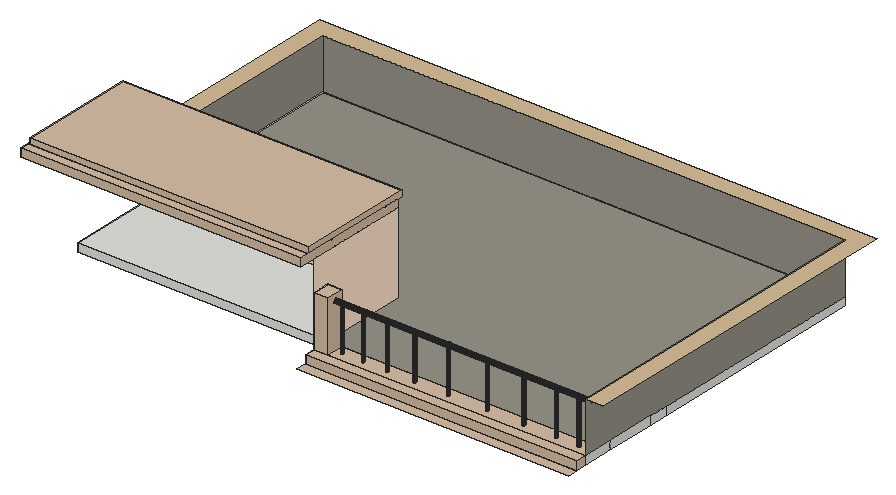
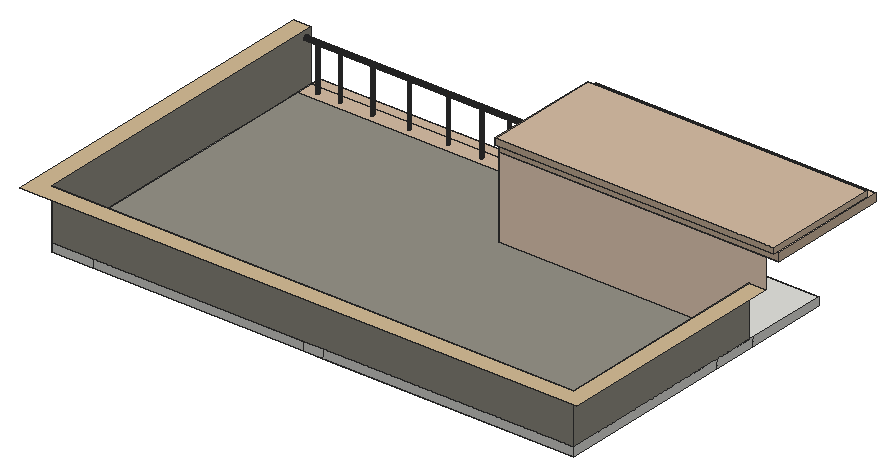
# SketchUp Ruby script. Lengths in inches.
U = 1.inch
M = Sketchup.active_model
def pt(a) = Geom::Point3d.new(a.map { |v| v * U })
def face(e, loops, mat)
  f = e.add_face(loops[0].map { |a| pt(a) })
  loops[1..].each { |l| e.add_face(l.map { |a| pt(a) }).erase! }
  f.material = f.back_material = mat if mat
  f
end
# faces: each face lists its corners as indices into pts; further lists are holes
def faces(e, pts, list, mat = nil) = list.each { |f| face(e, (f[0].is_a?(Array) ? f : [f]).map { |l| l.map { |i| pts[i] } }, mat) }
# xy, xz, yz: faces in a plane at the given z, y or x. An outline is a flat list of corners, or four numbers for a rectangle; further outlines are holes
def ring(l) = l.size == 4 ? [[l[0], l[1]], [l[2], l[1]], [l[2], l[3]], [l[0], l[3]]] : l.each_slice(2).to_a
def flat(e, list, mat, &to3) = list.each { |f| face(e, (f[0].is_a?(Array) ? f : [f]).map { |l| ring(l).map { |u, v| to3.(u, v) } }, mat) }
def xy(e, z, list, mat = nil) = flat(e, list, mat) { |x, y| [x, y, z] }
def xz(e, y, list, mat = nil) = flat(e, list, mat) { |x, z| [x, y, z] }
def yz(e, x, list, mat = nil) = flat(e, list, mat) { |y, z| [x, y, z] }
def lines(e, pts, list) = list.each { |a, b| e.add_line(pt(pts[a]), pt(pts[b])) }
# prism: a flat outline (further loops are holes) pulled along v
def prism(e, loops, v, mat = nil)
  f = face(e, loops, mat); d = Geom::Vector3d.new(v.map { |x| x * U })
  f.pushpull(f.normal.samedirection?(d) ? d.length : -d.length)
end
def box(e, o, s, mat = nil) = prism(e, [[o, [o[0] + s[0], o[1], o[2]], [o[0] + s[0], o[1] + s[1], o[2]], [o[0], o[1] + s[1], o[2]]]], [0, 0, s[2]], mat)
def at(x, y, z, deg = 0) = Geom::Transformation.translation(pt([x, y, z])) * Geom::Transformation.rotation(ORIGIN, Z_AXIS, deg.degrees)
def axes(o, x, y, z) = Geom::Transformation.new([*x, 0, *y, 0, *z, 0, *pt(o).to_a, 1])
def part(name) = M.definitions.add(name)
# library, detail: a bought-in or finely detailed component or shape, given as its bounding box
def library(name, o, s) = part(name).tap { |d| box(d.entities, o, s) }
def detail(e, o, s) = box(e.add_group.entities, o, s)
def put(e, d, t, mat = nil) = e.add_instance(d, t).tap { |i| i.material = mat if mat }
def group(e, t, mat = nil) = e.add_group.tap { |g| g.transformation = t; g.material = mat if mat }.entities
root = M.entities
M.materials.add("[Color C01]").color = [255, 229, 204]
M.materials.add("[Color C08]").color = [102, 51, 0]
M.materials.add("[Formica Beige]").color = [211, 187, 149]
M.materials.add("[Formica Graystone]").color = [149, 146, 135]
M.materials.add("[Formica Laminate Light]").color = [213, 189, 164]
xy(root,224.375,[[165.35,65.35,266.79,69.35],[71.76,75.87,165.35,106.73],[165.35,75.87,172.48,106.73],[172.48,75.87,187.4,80.84],[251.59,80.84,266.79,99.67],
  [172.48,88.8,187.4,99.67],[187.4,88.8,251.59,99.67],[172.48,99.67,251.59,106.73],[251.59,99.67,266.79,106.73],[71.76,106.73,165.35,123.48],
  [165.35,106.73,172.48,123.48],[172.48,106.73,251.59,190.6],[251.59,106.73,266.79,190.6],[71.76,123.48,165.35,190.6],[165.35,123.48,172.48,190.6]])
xy(root,224.375,[[165.35,61.48,266.79,65.35],[165.35,69.35,165.35,75.87,187.4,75.87,187.4,80.84,172.48,80.84,172.48,88.8,251.59,88.8,251.59,80.84,266.79,80.84,266.79,69.35]],"[Formica Laminate Light]")
xy(root,227.5,[[165.35,69.35,170.67,75.87],[173.23,72.18,173.1,72.19,172.98,72.24,172.88,72.32,172.8,72.43,172.75,72.55,172.73,72.68,172.75,72.81,172.8,72.93,172.88,73.03,172.98,73.11,173.1,73.16,173.23,73.18,173.36,73.16,173.48,73.11,173.58,73.03,173.66,72.93,173.71,72.81,173.73,72.68,173.71,72.55,173.66,72.43,173.58,72.32,173.48,72.24,173.36,72.19],[181.11,72.18,180.98,72.19,180.86,72.24,180.75,72.32,180.67,72.43,180.625,72.55,180.61,72.68,180.625,72.81,180.67,72.93,180.75,73.03,180.86,73.11,180.98,73.16,181.11,73.18,181.24,73.16,181.36,73.11,181.46,73.03,181.54,72.93,181.59,72.81,181.61,72.68,181.59,72.55,181.54,72.43,181.46,72.32,181.36,72.24,181.24,72.19],[190.17,72.18,190.04,72.19,189.92,72.24,189.81,72.32,189.74,72.43,189.6875,72.55,189.67,72.68,189.6875,72.81,189.74,72.93,189.81,73.03,189.92,73.11,190.04,73.16,190.17,73.18,190.3,73.16,190.42,73.11,190.52,73.03,190.6,72.93,190.65,72.81,190.67,72.68,190.65,72.55,190.6,72.43,190.52,72.32,190.42,72.24,190.3,72.19],[200.36,72.18,200.23,72.19,200.11,72.24,200,72.32,199.92,72.43,199.875,72.55,199.86,72.68,199.875,72.81,199.92,72.93,200,73.03,200.11,73.11,200.23,73.16,200.36,73.18,200.49,73.16,200.61,73.11,200.71,73.03,200.79,72.93,200.84,72.81,200.86,72.68,200.84,72.55,200.79,72.43,200.71,72.32,200.61,72.24,200.49,72.19],
  [212.98,72.18,212.85,72.19,212.73,72.24,212.63,72.32,212.55,72.43,212.5,72.55,212.48,72.68,212.5,72.81,212.55,72.93,212.63,73.03,212.73,73.11,212.85,73.16,212.98,73.18,213.11,73.16,213.23,73.11,213.33,73.03,213.41,72.93,213.46,72.81,213.48,72.68,213.46,72.55,213.41,72.43,213.33,72.32,213.23,72.24,213.11,72.19],[227.42,72.18,227.29,72.19,227.17,72.24,227.06,72.32,226.99,72.43,226.9375,72.55,226.92,72.68,226.9375,72.81,226.99,72.93,227.06,73.03,227.17,73.11,227.29,73.16,227.42,73.18,227.55,73.16,227.67,73.11,227.77,73.03,227.85,72.93,227.9,72.81,227.92,72.68,227.9,72.55,227.85,72.43,227.77,72.32,227.67,72.24,227.55,72.19],[241.17,72.18,241.04,72.19,240.92,72.24,240.81,72.32,240.74,72.43,240.6875,72.55,240.67,72.68,240.6875,72.81,240.74,72.93,240.81,73.03,240.92,73.11,241.04,73.16,241.17,73.18,241.3,73.16,241.42,73.11,241.52,73.03,241.6,72.93,241.65,72.81,241.67,72.68,241.65,72.55,241.6,72.43,241.52,72.32,241.42,72.24,241.3,72.19],[253.36,72.18,253.23,72.19,253.11,72.24,253,72.32,252.92,72.43,252.875,72.55,252.86,72.68,252.875,72.81,252.92,72.93,253,73.03,253.11,73.11,253.23,73.16,253.36,73.18,253.49,73.16,253.61,73.11,253.71,73.03,253.79,72.93,253.84,72.81,253.86,72.68,253.84,72.55,253.79,72.43,253.71,72.32,253.61,72.24,253.49,72.19],[261.73,72.18,261.6,72.19,261.48,72.24,261.38,72.32,261.3,72.43,261.25,72.55,261.23,72.68,261.25,72.81,261.3,72.93,261.38,73.03,261.48,73.11,261.6,73.16,261.73,73.18,261.86,73.16,261.98,73.11,262.08,73.03,262.16,72.93,262.21,72.81,262.23,72.68,262.21,72.55,262.16,72.43,262.08,72.32,261.98,72.24,261.86,72.19],
  [71.76,75.87,165.35,108.74]])
xy(root,227.5,[[165.35,75.87,266.79,75.87,266.79,190.6,71.76,190.6,71.76,108.74,165.35,108.74]],"[Formica Graystone]")
xy(root,227.5,[[165.35,65.35,266.79,69.35],[[170.67,69.35,266.79,75.87],[261.73,72.18,261.6,72.19,261.48,72.24,261.38,72.32,261.3,72.43,261.25,72.55,261.23,72.68,261.25,72.81,261.3,72.93,261.38,73.03,261.48,73.11,261.6,73.16,261.73,73.18,261.86,73.16,261.98,73.11,262.08,73.03,262.16,72.93,262.21,72.81,262.23,72.68,262.21,72.55,262.16,72.43,262.08,72.32,261.98,72.24,261.86,72.19],[173.23,72.18,173.1,72.19,172.98,72.24,172.88,72.32,172.8,72.43,172.75,72.55,172.73,72.68,172.75,72.81,172.8,72.93,172.88,73.03,172.98,73.11,173.1,73.16,173.23,73.18,173.36,73.16,173.48,73.11,173.58,73.03,173.66,72.93,173.71,72.81,173.73,72.68,173.71,72.55,173.66,72.43,173.58,72.32,173.48,72.24,173.36,72.19],[181.11,72.18,180.98,72.19,180.86,72.24,180.75,72.32,180.67,72.43,180.625,72.55,180.61,72.68,180.625,72.81,180.67,72.93,180.75,73.03,180.86,73.11,180.98,73.16,181.11,73.18,181.24,73.16,181.36,73.11,181.46,73.03,181.54,72.93,181.59,72.81,181.61,72.68,181.59,72.55,181.54,72.43,181.46,72.32,181.36,72.24,181.24,72.19],[253.36,72.18,253.23,72.19,253.11,72.24,253,72.32,252.92,72.43,252.875,72.55,252.86,72.68,252.875,72.81,252.92,72.93,253,73.03,253.11,73.11,253.23,73.16,253.36,73.18,253.49,73.16,253.61,73.11,253.71,73.03,253.79,72.93,253.84,72.81,253.86,72.68,253.84,72.55,253.79,72.43,253.71,72.32,253.61,72.24,253.49,72.19],[190.17,72.18,190.04,72.19,189.92,72.24,189.81,72.32,189.74,72.43,189.6875,72.55,189.67,72.68,189.6875,72.81,189.74,72.93,189.81,73.03,189.92,73.11,190.04,73.16,190.17,73.18,190.3,73.16,190.42,73.11,190.52,73.03,190.6,72.93,190.65,72.81,190.67,72.68,190.65,72.55,190.6,72.43,190.52,72.32,190.42,72.24,190.3,72.19],[241.17,72.18,241.04,72.19,240.92,72.24,240.81,72.32,240.74,72.43,240.6875,72.55,240.67,72.68,240.6875,72.81,240.74,72.93,240.81,73.03,240.92,73.11,241.04,73.16,241.17,73.18,241.3,73.16,241.42,73.11,241.52,73.03,241.6,72.93,241.65,72.81,241.67,72.68,241.65,72.55,241.6,72.43,241.52,72.32,241.42,72.24,241.3,72.19],[200.36,72.18,200.23,72.19,200.11,72.24,200,72.32,199.92,72.43,199.875,72.55,199.86,72.68,199.875,72.81,199.92,72.93,200,73.03,200.11,73.11,200.23,73.16,200.36,73.18,200.49,73.16,200.61,73.11,200.71,73.03,200.79,72.93,200.84,72.81,200.86,72.68,200.84,72.55,200.79,72.43,200.71,72.32,200.61,72.24,200.49,72.19],[227.42,72.18,227.29,72.19,227.17,72.24,227.06,72.32,226.99,72.43,226.9375,72.55,226.92,72.68,226.9375,72.81,226.99,72.93,227.06,73.03,227.17,73.11,227.29,73.16,227.42,73.18,227.55,73.16,227.67,73.11,227.77,73.03,227.85,72.93,227.9,72.81,227.92,72.68,227.9,72.55,227.85,72.43,227.77,72.32,227.67,72.24,227.55,72.19],[212.98,72.18,212.85,72.19,212.73,72.24,212.63,72.32,212.55,72.43,212.5,72.55,212.48,72.68,212.5,72.81,212.55,72.93,212.63,73.03,212.73,73.11,212.85,73.16,212.98,73.18,213.11,73.16,213.23,73.11,213.33,73.03,213.41,72.93,213.46,72.81,213.48,72.68,213.46,72.55,213.41,72.43,213.33,72.32,213.23,72.24,213.11,72.19]]],"[Formica Laminate Light]")
xy(root,244.1875,[[261.73,72.18,261.86,72.19,261.98,72.24,262.08,72.32,262.16,72.43,262.21,72.55,262.23,72.68,262.21,72.81,262.16,72.93,262.08,73.03,261.98,73.11,261.86,73.16,261.73,73.18,261.6,73.16,261.48,73.11,261.38,73.03,261.3,72.93,261.25,72.81,261.23,72.68,261.25,72.55,261.3,72.43,261.38,72.32,261.48,72.24,261.6,72.19]])
xy(root,244.3125,[[200.36,72.18,200.49,72.19,200.61,72.24,200.71,72.32,200.79,72.43,200.84,72.55,200.86,72.68,200.84,72.81,200.79,72.93,200.71,73.03,200.61,73.11,200.49,73.16,200.36,73.18,200.23,73.16,200.11,73.11,200,73.03,199.92,72.93,199.875,72.81,199.86,72.68,199.875,72.55,199.92,72.43,200,72.32,200.11,72.24,200.23,72.19]])
xy(root,244.38,[[173.23,72.18,173.36,72.19,173.48,72.24,173.58,72.32,173.66,72.43,173.71,72.55,173.73,72.68,173.71,72.81,173.66,72.93,173.58,73.03,173.48,73.11,173.42,73.13,173.04,73.13,172.98,73.11,172.88,73.03,172.8,72.93,172.75,72.81,172.73,72.68,172.75,72.55,172.8,72.43,172.88,72.32,172.98,72.24,173.1,72.19],[173.04,73.13,173.42,73.13,173.36,73.16,173.23,73.18,173.1,73.16]])
xy(root,244.4375,[[181.11,72.18,181.24,72.19,181.36,72.24,181.46,72.32,181.54,72.43,181.59,72.55,181.61,72.68,181.59,72.81,181.54,72.93,181.46,73.03,181.36,73.11,181.24,73.16,181.11,73.18,180.98,73.16,180.86,73.11,180.75,73.03,180.67,72.93,180.625,72.81,180.61,72.68,180.625,72.55,180.67,72.43,180.75,72.32,180.86,72.24,180.98,72.19]])
xy(root,244.5,[[190.17,72.18,190.3,72.19,190.42,72.24,190.52,72.32,190.6,72.43,190.65,72.55,190.67,72.68,190.65,72.81,190.6,72.93,190.52,73.03,190.42,73.11,190.3,73.16,190.17,73.18,190.04,73.16,189.92,73.11,189.81,73.03,189.74,72.93,189.6875,72.81,189.67,72.68,189.6875,72.55,189.74,72.43,189.81,72.32,189.92,72.24,190.04,72.19],[241.17,72.18,241.3,72.19,241.42,72.24,241.52,72.32,241.6,72.43,241.65,72.55,241.67,72.68,241.65,72.81,241.6,72.93,241.52,73.03,241.42,73.11,241.3,73.16,241.17,73.18,241.04,73.16,240.92,73.11,240.81,73.03,240.74,72.93,240.6875,72.81,240.67,72.68,240.6875,72.55,240.74,72.43,240.81,72.32,240.92,72.24,241.04,72.19]])
xy(root,244.56,[[227.42,72.18,227.55,72.19,227.67,72.24,227.77,72.32,227.85,72.43,227.9,72.55,227.92,72.68,227.9,72.81,227.85,72.93,227.77,73.03,227.67,73.11,227.17,73.11,227.06,73.03,226.99,72.93,226.9375,72.81,226.92,72.68,226.9375,72.55,226.99,72.43,227.06,72.32,227.17,72.24,227.29,72.19],[227.17,73.11,227.67,73.11,227.55,73.16,227.42,73.18,227.29,73.16]])
xy(root,244.5625,[[253.36,72.18,253.49,72.19,253.61,72.24,253.71,72.32,253.79,72.43,253.84,72.55,253.86,72.68,253.84,72.81,253.79,72.93,253.71,73.03,253.61,73.11,253.49,73.16,253.36,73.18,253.23,73.16,253.11,73.11,253,73.03,252.92,72.93,252.875,72.81,252.86,72.68,252.875,72.55,252.92,72.43,253,72.32,253.11,72.24,253.23,72.19]])
xy(root,244.9375,[[212.98,72.18,213.11,72.19,213.23,72.24,213.33,72.32,213.41,72.43,213.46,72.55,213.48,72.68,213.46,72.81,213.41,72.93,213.33,73.03,213.23,73.11,213.11,73.16,212.98,73.18,212.85,73.16,212.73,73.11,212.63,73.03,212.55,72.93,212.5,72.81,212.48,72.68,212.5,72.55,212.55,72.43,212.63,72.32,212.73,72.24,212.85,72.19]])
xy(root,246.5,[[266.79,69.35,273.31,69.35,273.31,197.12,65.24,197.12,65.24,108.74,71.76,108.74,71.76,190.6,266.79,190.6]],"[Formica Beige]")
xy(root,246.5,[[165.35,69.35,170.67,75.87]],"[Formica Laminate Light]")
xy(root,257.76,[[65.24,69.35,165.35,108.74]])
xy(root,257.76,[[60.43,63.29,60.43,108.74,65.24,108.74,65.24,69.35,165.35,69.35,165.35,63.29]],"[Formica Laminate Light]")
xy(root,260.6875,[[61.24,66.91,165.35,108.74],[61.24,108.74,165.35,110.3]])
xy(root,260.6875,[[60.43,63.29,165.35,66.91],[60.43,66.91,61.24,108.74]],"[Formica Laminate Light]")
xy(root,262.8125,[[61.24,66.91,165.35,110.3]],"[Formica Laminate Light]")
xz(root,63.29,[[60.43,257.76,165.35,260.6875]],"[Formica Laminate Light]")
xz(root,65.35,[[165.35,224.375,266.79,227.5]],"[Formica Laminate Light]")
xz(root,66.91,[[61.24,260.6875,165.35,262.8125]],"[Formica Laminate Light]")
xz(root,69.35,[[165.35,227.5,170.67,246.5]],"[Formica Laminate Light]")
xz(root,75.87,[[71.76,224.375,165.35,227.5]])
xz(root,75.87,[[165.35,227.5,170.67,246.5]],"[Formica Laminate Light]")
xz(root,108.74,[[71.76,227.5,71.76,246.5,65.24,246.5,65.24,257.76,165.35,257.76,165.35,227.5]],"[Color C01]")
xz(root,108.74,[[60.43,257.76,165.35,260.6875]],"[Formica Laminate Light]")
xz(root,110.3,[[61.24,260.6875,165.35,262.8125]],"[Formica Laminate Light]")
xz(root,190.6,[[71.76,224.375,165.35,227.5],[165.35,224.375,172.48,227.5],[172.48,224.375,251.59,227.5],[251.59,224.375,266.79,227.5]])
xz(root,190.6,[[71.76,227.5,266.79,246.5]],"[Formica Graystone]")
yz(root,60.43,[[63.29,257.76,108.74,260.6875]],"[Formica Laminate Light]")
yz(root,61.24,[[66.91,260.6875,110.3,262.8125]],"[Formica Laminate Light]")
yz(root,71.76,[[75.87,224.375,106.73,227.5],[106.73,224.375,123.48,227.5],[123.48,224.375,190.6,227.5]])
yz(root,71.76,[[108.74,227.5,190.6,246.5]],"[Formica Graystone]")
yz(root,165.35,[[69.35,224.375,75.87,227.5],[69.35,227.5,75.87,246.5]])
yz(root,165.35,[[75.87,227.5,108.74,227.5,108.74,257.76,69.35,257.76,69.35,246.5,75.87,246.5]],"[Color C01]")
yz(root,165.35,[[65.35,224.375,69.35,227.5],[63.29,257.76,108.74,260.6875],[66.91,260.6875,110.3,262.8125]],"[Formica Laminate Light]")
yz(root,170.67,[[72.44,243.69,72.27,243.72,72.1,243.79,71.96,243.89,71.85,244.04,71.78,244.2,71.76,244.38,71.78,244.56,71.85,244.72,71.96,244.87,72.1,244.98,72.27,245.04,72.44,245.07,72.62,245.04,72.79,244.98,72.93,244.87,73.04,244.72,73.11,244.56,73.13,244.38,73.11,244.2,73.04,244.04,72.93,243.89,72.79,243.79,72.62,243.72]])
yz(root,170.67,[[[69.35,227.5,75.87,246.5],[72.44,243.69,72.27,243.72,72.1,243.79,71.96,243.89,71.85,244.04,71.78,244.2,71.76,244.38,71.78,244.56,71.85,244.72,71.96,244.87,72.1,244.98,72.27,245.04,72.44,245.07,72.62,245.04,72.79,244.98,72.93,244.87,73.04,244.72,73.11,244.56,73.13,244.38,73.11,244.2,73.04,244.04,72.93,243.89,72.79,243.79,72.62,243.72]]],"[Formica Laminate Light]")
yz(root,266.79,[[69.35,224.375,80.84,227.5],[80.84,224.375,99.67,227.5],[99.67,224.375,106.73,227.5],[106.73,224.375,190.6,227.5]])
yz(root,266.79,[[[69.35,227.5,190.6,246.5],[72.44,243.69,72.62,243.72,72.79,243.79,72.93,243.89,73.04,244.04,73.11,244.2,73.13,244.38,73.11,244.56,73.04,244.72,72.93,244.87,72.79,244.98,72.62,245.04,72.44,245.07,72.27,245.04,72.1,244.98,71.96,244.87,71.85,244.72,71.78,244.56,71.76,244.38,71.78,244.2,71.85,244.04,71.96,243.89,72.1,243.79,72.27,243.72]]],"[Formica Graystone]")
yz(root,266.79,[[65.35,224.375,69.35,227.5]],"[Formica Laminate Light]")
p = [[172.88,72.32,227.5],[172.98,72.24,227.5],[172.98,72.24,244.38],[172.88,72.32,244.38],[173.1,72.19,227.5],[173.1,72.19,244.38],
  [173.23,72.18,227.5],[173.23,72.18,244.38],[173.36,72.19,227.5],[173.36,72.19,244.38],[173.48,72.24,227.5],[173.48,72.24,244.38],
  [173.58,72.32,227.5],[173.58,72.32,244.38],[180.75,72.32,227.5],[180.86,72.24,227.5],[180.86,72.24,244.4375],[180.75,72.32,244.4375],
  [180.98,72.19,227.5],[180.98,72.19,244.4375],[181.11,72.18,227.5],[181.11,72.18,244.4375],[181.24,72.19,227.5],[181.24,72.19,244.4375],
  [181.36,72.24,227.5],[181.36,72.24,244.4375],[181.46,72.32,227.5],[181.46,72.32,244.4375],[189.81,72.32,227.5],[189.92,72.24,227.5],
  [189.92,72.24,244.5],[189.81,72.32,244.5],[190.04,72.19,227.5],[190.04,72.19,244.5],[190.17,72.18,227.5],[190.17,72.18,244.5],
  [190.3,72.19,227.5],[190.3,72.19,244.5],[190.42,72.24,227.5],[190.42,72.24,244.5],[190.52,72.32,227.5],[190.52,72.32,244.5],
  [200,72.32,227.5],[200.11,72.24,227.5],[200.11,72.24,244.3125],[200,72.32,244.3125],[200.23,72.19,227.5],[200.23,72.19,244.3125],
  [200.36,72.18,227.5],[200.36,72.18,244.3125],[200.49,72.19,227.5],[200.49,72.19,244.3125],[200.61,72.24,227.5],[200.61,72.24,244.3125],
  [200.71,72.32,227.5],[200.71,72.32,244.3125],[212.63,72.32,227.5],[212.73,72.24,227.5],[212.73,72.24,244.9375],[212.63,72.32,244.9375],
  [212.85,72.19,227.5],[212.85,72.19,244.9375],[212.98,72.18,227.5],[212.98,72.18,244.9375],[213.11,72.19,227.5],[213.11,72.19,244.9375],
  [213.23,72.24,227.5],[213.23,72.24,244.9375],[213.33,72.32,227.5],[213.33,72.32,244.9375],[227.06,72.32,227.5],[227.17,72.24,227.5],
  [227.17,72.24,244.56],[227.06,72.32,244.56],[227.29,72.19,227.5],[227.29,72.19,244.56],[227.42,72.18,227.5],[227.42,72.18,244.56],
  [227.55,72.19,227.5],[227.55,72.19,244.56],[227.67,72.24,227.5],[227.67,72.24,244.56],[227.77,72.32,227.5],[227.77,72.32,244.56],
  [240.81,72.32,227.5],[240.92,72.24,227.5],[240.92,72.24,244.5],[240.81,72.32,244.5],[241.04,72.19,227.5],[241.04,72.19,244.5],
  [241.17,72.18,227.5],[241.17,72.18,244.5],[241.3,72.19,227.5],[241.3,72.19,244.5],[241.42,72.24,227.5],[241.42,72.24,244.5],
  [241.52,72.32,227.5],[241.52,72.32,244.5],[253,72.32,227.5],[253.11,72.24,227.5],[253.11,72.24,244.5625],[253,72.32,244.5625],
  [253.23,72.19,227.5],[253.23,72.19,244.5625],[253.36,72.18,227.5],[253.36,72.18,244.5625],[253.49,72.19,227.5],[253.49,72.19,244.5625],
  [253.61,72.24,227.5],[253.61,72.24,244.5625],[253.71,72.32,227.5],[253.71,72.32,244.5625],[261.38,72.32,227.5],[261.48,72.24,227.5],
  [261.48,72.24,244.1875],[261.38,72.32,244.1875],[261.6,72.19,227.5],[261.6,72.19,244.1875],[261.73,72.18,227.5],[261.73,72.18,244.1875],
  [261.86,72.19,227.5],[261.86,72.19,244.1875],[261.98,72.24,227.5],[261.98,72.24,244.1875],[262.08,72.32,227.5],[262.08,72.32,244.1875],
  [172.8,72.43,227.5],[172.8,72.43,244.38],[173.66,72.43,227.5],[173.66,72.43,244.38],[180.67,72.43,227.5],[180.67,72.43,244.4375],
  [181.54,72.43,227.5],[181.54,72.43,244.4375],[189.74,72.43,227.5],[189.74,72.43,244.5],[190.6,72.43,227.5],[190.6,72.43,244.5],
  [199.92,72.43,227.5],[199.92,72.43,244.3125],[200.79,72.43,227.5],[200.79,72.43,244.3125],[212.55,72.43,227.5],[212.55,72.43,244.9375],
  [213.41,72.43,227.5],[213.41,72.43,244.9375],[226.99,72.43,227.5],[226.99,72.43,244.56],[227.85,72.43,227.5],[227.85,72.43,244.56],
  [240.74,72.43,227.5],[240.74,72.43,244.5],[241.6,72.43,227.5],[241.6,72.43,244.5],[252.92,72.43,227.5],[252.92,72.43,244.5625],
  [253.79,72.43,227.5],[253.79,72.43,244.5625],[261.3,72.43,227.5],[261.3,72.43,244.1875],[262.16,72.43,227.5],[262.16,72.43,244.1875],
  [172.75,72.55,227.5],[172.75,72.55,244.38],[173.71,72.55,227.5],[173.71,72.55,244.38],[180.625,72.55,227.5],[180.625,72.55,244.4375],
  [181.59,72.55,227.5],[181.59,72.55,244.4375],[189.6875,72.55,227.5],[189.6875,72.55,244.5],[190.65,72.55,227.5],[190.65,72.55,244.5],
  [199.875,72.55,227.5],[199.875,72.55,244.3125],[200.84,72.55,227.5],[200.84,72.55,244.3125],[212.5,72.55,227.5],[212.5,72.55,244.9375],
  [213.46,72.55,227.5],[213.46,72.55,244.9375],[226.9375,72.55,227.5],[226.9375,72.55,244.56],[227.9,72.55,227.5],[227.9,72.55,244.56],
  [240.6875,72.55,227.5],[240.6875,72.55,244.5],[241.65,72.55,227.5],[241.65,72.55,244.5],[252.875,72.55,227.5],[252.875,72.55,244.5625],
  [253.84,72.55,227.5],[253.84,72.55,244.5625],[261.25,72.55,227.5],[261.25,72.55,244.1875],[262.21,72.55,227.5],[262.21,72.55,244.1875],
  [172.73,72.68,227.5],[172.73,72.68,244.38],[173.73,72.68,227.5],[173.73,72.68,244.38],[180.61,72.68,227.5],[180.61,72.68,244.4375],
  [181.61,72.68,227.5],[181.61,72.68,244.4375],[189.67,72.68,227.5],[189.67,72.68,244.5],[190.67,72.68,227.5],[190.67,72.68,244.5],
  [199.86,72.68,227.5],[199.86,72.68,244.3125],[200.86,72.68,227.5],[200.86,72.68,244.3125],[212.48,72.68,227.5],[212.48,72.68,244.9375],
  [213.48,72.68,227.5],[213.48,72.68,244.9375],[226.92,72.68,227.5],[226.92,72.68,244.56],[227.92,72.68,227.5],[227.92,72.68,244.56],
  [240.67,72.68,227.5],[240.67,72.68,244.5],[241.67,72.68,227.5],[241.67,72.68,244.5],[252.86,72.68,227.5],[252.86,72.68,244.5625],
  [253.86,72.68,227.5],[253.86,72.68,244.5625],[261.23,72.68,227.5],[261.23,72.68,244.1875],[262.23,72.68,227.5],[262.23,72.68,244.1875],
  [172.75,72.81,227.5],[172.75,72.81,244.38],[173.71,72.81,227.5],[173.71,72.81,244.38],[180.625,72.81,227.5],[180.625,72.81,244.4375],
  [181.59,72.81,227.5],[181.59,72.81,244.4375],[189.6875,72.81,227.5],[189.6875,72.81,244.5],[190.65,72.81,227.5],[190.65,72.81,244.5],
  [199.875,72.81,227.5],[199.875,72.81,244.3125],[200.84,72.81,227.5],[200.84,72.81,244.3125],[212.5,72.81,227.5],[212.5,72.81,244.9375],
  [213.46,72.81,227.5],[213.46,72.81,244.9375],[226.9375,72.81,227.5],[226.9375,72.81,244.56],[227.9,72.81,227.5],[227.9,72.81,244.56],
  [240.6875,72.81,227.5],[240.6875,72.81,244.5],[241.65,72.81,227.5],[241.65,72.81,244.5],[252.875,72.81,227.5],[252.875,72.81,244.5625],
  [253.84,72.81,227.5],[253.84,72.81,244.5625],[261.25,72.81,227.5],[261.25,72.81,244.1875],[262.21,72.81,227.5],[262.21,72.81,244.1875],
  [172.8,72.93,227.5],[172.8,72.93,244.38],[173.66,72.93,227.5],[173.66,72.93,244.38],[180.67,72.93,227.5],[180.67,72.93,244.4375],
  [181.54,72.93,227.5],[181.54,72.93,244.4375],[189.74,72.93,227.5],[189.74,72.93,244.5],[190.6,72.93,227.5],[190.6,72.93,244.5],
  [199.92,72.93,227.5],[199.92,72.93,244.3125],[200.79,72.93,227.5],[200.79,72.93,244.3125],[212.55,72.93,227.5],[212.55,72.93,244.9375],
  [213.41,72.93,227.5],[213.41,72.93,244.9375],[226.99,72.93,227.5],[226.99,72.93,244.56],[227.85,72.93,227.5],[227.85,72.93,244.56],
  [240.74,72.93,227.5],[240.74,72.93,244.5],[241.6,72.93,227.5],[241.6,72.93,244.5],[252.92,72.93,227.5],[252.92,72.93,244.5625],
  [253.79,72.93,227.5],[253.79,72.93,244.5625],[261.3,72.93,227.5],[261.3,72.93,244.1875],[262.16,72.93,227.5],[262.16,72.93,244.1875],
  [172.88,73.03,227.5],[172.88,73.03,244.38],[173.58,73.03,227.5],[173.58,73.03,244.38],[180.75,73.03,227.5],[180.75,73.03,244.4375],
  [181.46,73.03,227.5],[181.46,73.03,244.4375],[189.81,73.03,227.5],[189.81,73.03,244.5],[190.52,73.03,227.5],[190.52,73.03,244.5],
  [200,73.03,227.5],[200,73.03,244.3125],[200.71,73.03,227.5],[200.71,73.03,244.3125],[212.63,73.03,227.5],[212.63,73.03,244.9375],
  [213.33,73.03,227.5],[213.33,73.03,244.9375],[227.06,73.03,227.5],[227.06,73.03,244.56],[227.77,73.03,227.5],[227.77,73.03,244.56],
  [240.81,73.03,227.5],[240.81,73.03,244.5],[241.52,73.03,227.5],[241.52,73.03,244.5],[253,73.03,227.5],[253,73.03,244.5625],
  [253.71,73.03,227.5],[253.71,73.03,244.5625],[261.38,73.03,227.5],[261.38,73.03,244.1875],[262.08,73.03,227.5],[262.08,73.03,244.1875],
  [172.98,73.11,227.5],[172.98,73.11,244.38],[172.98,73.11,244.2],[173.48,73.11,227.5],[173.48,73.11,244.2],[173.48,73.11,244.38],
  [180.86,73.11,227.5],[180.86,73.11,244.4375],[180.86,73.11,244.2],[181.36,73.11,227.5],[181.36,73.11,244.2],[181.36,73.11,244.4375],
  [189.92,73.11,227.5],[189.92,73.11,244.5],[189.92,73.11,244.2],[190.42,73.11,227.5],[190.42,73.11,244.2],[190.42,73.11,244.5],
  [200.11,73.11,227.5],[200.11,73.11,244.3125],[200.11,73.11,244.2],[200.61,73.11,227.5],[200.61,73.11,244.2],[200.61,73.11,244.3125],
  [212.73,73.11,227.5],[212.73,73.11,244.9375],[212.73,73.11,244.56],[212.73,73.11,244.2],[213.23,73.11,227.5],[213.23,73.11,244.2],
  [213.23,73.11,244.56],[213.23,73.11,244.9375],[227.17,73.11,227.5],[227.17,73.11,244.56],[227.17,73.11,244.2],[227.67,73.11,227.5],
  [227.67,73.11,244.2],[227.67,73.11,244.56],[240.92,73.11,227.5],[240.92,73.11,244.5],[240.92,73.11,244.2],[241.42,73.11,227.5],
  [241.42,73.11,244.2],[241.42,73.11,244.5],[253.11,73.11,227.5],[253.11,73.11,244.5625],[253.11,73.11,244.56],[253.11,73.11,244.2],
  [253.61,73.11,227.5],[253.61,73.11,244.2],[253.61,73.11,244.56],[253.61,73.11,244.5625],[261.48,73.11,227.5],[261.48,73.11,244.1875],
  [261.98,73.11,227.5],[261.98,73.11,244.1875],[173.1,73.16,227.5],[173.04,73.13,244.38],[173.1,73.16,244.38],[173.36,73.16,227.5],
  [173.36,73.16,244.38],[173.42,73.13,244.38],[180.98,73.16,227.5],[180.98,73.16,244.4375],[181.24,73.16,227.5],[181.24,73.16,244.4375],
  [190.04,73.16,227.5],[190.04,73.16,244.5],[190.3,73.16,227.5],[190.3,73.16,244.5],[200.23,73.16,227.5],[200.23,73.16,244.3125],
  [200.49,73.16,227.5],[200.49,73.16,244.3125],[212.85,73.16,227.5],[212.85,73.16,244.9375],[213.11,73.16,227.5],[213.11,73.16,244.9375],
  [227.29,73.16,227.5],[227.29,73.16,244.56],[227.55,73.16,227.5],[227.55,73.16,244.56],[241.04,73.16,227.5],[241.04,73.16,244.5],
  [241.3,73.16,227.5],[241.3,73.16,244.5],[253.23,73.16,227.5],[253.23,73.16,244.5625],[253.49,73.16,227.5],[253.49,73.16,244.5625],
  [261.6,73.16,227.5],[261.6,73.16,244.1875],[261.86,73.16,227.5],[261.86,73.16,244.1875],[173.23,73.18,227.5],[173.23,73.18,244.38],
  [181.11,73.18,227.5],[181.11,73.18,244.4375],[190.17,73.18,227.5],[190.17,73.18,244.5],[200.36,73.18,227.5],[200.36,73.18,244.3125],
  [212.98,73.18,227.5],[212.98,73.18,244.9375],[227.42,73.18,227.5],[227.42,73.18,244.56],[241.17,73.18,227.5],[241.17,73.18,244.5],
  [253.36,73.18,227.5],[253.36,73.18,244.5625],[261.73,73.18,227.5],[261.73,73.18,244.1875],[170.67,72.1,243.79],[170.67,72.27,243.72],
  [266.79,72.27,243.72],[266.79,72.1,243.79],[170.67,72.44,243.69],[266.79,72.44,243.69],[170.67,72.62,243.72],[266.79,72.62,243.72],
  [170.67,72.79,243.79],[266.79,72.79,243.79],[170.67,71.96,243.89],[266.79,71.96,243.89],[170.67,72.93,243.89],[266.79,72.93,243.89],
  [170.67,71.85,244.04],[266.79,71.85,244.04],[170.67,73.04,244.04],[266.79,73.04,244.04],[170.67,71.78,244.2],[266.79,71.78,244.2],
  [170.67,73.11,244.2],[266.79,73.11,244.2],[170.67,71.76,244.38],[266.79,71.76,244.38],[170.67,73.13,244.38],[266.79,73.13,244.38],
  [170.67,71.78,244.56],[266.79,71.78,244.56],[170.67,73.11,244.56],[266.79,73.11,244.56],[170.67,71.85,244.72],[266.79,71.85,244.72],
  [170.67,73.04,244.72],[266.79,73.04,244.72],[170.67,71.96,244.87],[266.79,71.96,244.87],[170.67,72.93,244.87],[266.79,72.93,244.87],
  [170.67,72.1,244.98],[266.79,72.1,244.98],[170.67,72.79,244.98],[266.79,72.79,244.98],[170.67,72.27,245.04],[266.79,72.27,245.04],
  [170.67,72.44,245.07],[266.79,72.44,245.07],[170.67,72.62,245.04],[266.79,72.62,245.04]]
faces(root,p,[[0,1,2,3],[1,4,5,2],[4,6,7,5],[6,8,9,7],[8,10,11,9],[10,12,13,11],[14,15,16,17],[15,18,19,16],
  [18,20,21,19],[20,22,23,21],[22,24,25,23],[24,26,27,25],[28,29,30,31],[29,32,33,30],[32,34,35,33],[34,36,37,35],
  [36,38,39,37],[38,40,41,39],[42,43,44,45],[43,46,47,44],[46,48,49,47],[48,50,51,49],[50,52,53,51],[52,54,55,53],
  [56,57,58,59],[57,60,61,58],[60,62,63,61],[62,64,65,63],[64,66,67,65],[66,68,69,67],[70,71,72,73],[71,74,75,72],
  [74,76,77,75],[76,78,79,77],[78,80,81,79],[80,82,83,81],[84,85,86,87],[85,88,89,86],[88,90,91,89],[90,92,93,91],
  [92,94,95,93],[94,96,97,95],[98,99,100,101],[99,102,103,100],[102,104,105,103],[104,106,107,105],[106,108,109,107],[108,110,111,109],
  [112,113,114,115],[113,116,117,114],[116,118,119,117],[118,120,121,119],[120,122,123,121],[122,124,125,123],[126,0,3,127],[12,128,129,13],
  [130,14,17,131],[26,132,133,27],[134,28,31,135],[40,136,137,41],[138,42,45,139],[54,140,141,55],[142,56,59,143],[68,144,145,69],
  [146,70,73,147],[82,148,149,83],[150,84,87,151],[96,152,153,97],[154,98,101,155],[110,156,157,111],[158,112,115,159],[124,160,161,125],
  [162,126,127,163],[128,164,165,129],[166,130,131,167],[132,168,169,133],[170,134,135,171],[136,172,173,137],[174,138,139,175],[140,176,177,141],
  [178,142,143,179],[144,180,181,145],[182,146,147,183],[148,184,185,149],[186,150,151,187],[152,188,189,153],[190,154,155,191],[156,192,193,157],
  [194,158,159,195],[160,196,197,161],[198,162,163,199],[164,200,201,165],[202,166,167,203],[168,204,205,169],[206,170,171,207],[172,208,209,173],
  [210,174,175,211],[176,212,213,177],[214,178,179,215],[180,216,217,181],[218,182,183,219],[184,220,221,185],[222,186,187,223],[188,224,225,189],
  [226,190,191,227],[192,228,229,193],[230,194,195,231],[196,232,233,197],[234,198,199,235],[200,236,237,201],[238,202,203,239],[204,240,241,205],
  [242,206,207,243],[208,244,245,209],[246,210,211,247],[212,248,249,213],[250,214,215,251],[216,252,253,217],[254,218,219,255],[220,256,257,221],
  [258,222,223,259],[224,260,261,225],[262,226,227,263],[228,264,265,229],[266,230,231,267],[232,268,269,233],[270,234,235,271],[236,272,273,237],
  [274,238,239,275],[240,276,277,241],[278,242,243,279],[244,280,281,245],[282,246,247,283],[248,284,285,249],[286,250,251,287],[252,288,289,253],
  [290,254,255,291],[256,292,293,257],[294,258,259,295],[260,296,297,261],[298,262,263,299],[264,300,301,265],[302,266,267,303],[268,304,305,269],
  [306,270,271,307],[272,308,309,273],[310,274,275,311],[276,312,313,277],[314,278,279,315],[280,316,317,281],[318,282,283,319],[284,320,321,285],
  [322,286,287,323],[288,324,325,289],[326,290,291,327],[292,328,329,293],[330,294,295,331],[296,332,333,297],[334,298,299,335],[300,336,337,301],
  [338,302,303,339],[304,340,341,305],[342,306,307,343,344],[308,345,346,347,309],[348,310,311,349,350],[312,351,352,353,313],[354,314,315,355,356],[316,357,358,359,317],
  [360,318,319,361,362],[320,363,364,365,321],[366,322,323,367,368,369],[324,370,371,372,373,325],[374,326,327,375,376],[328,377,378,379,329],[380,330,331,381,382],[332,383,384,385,333],
  [386,334,335,387,388,389],[336,390,391,392,393,337],[394,338,339,395],[340,396,397,341],[398,342,344,343,399,400],[345,401,402,403,347,346],[404,348,350,349,405],[351,406,407,353,352],
  [408,354,356,355,409],[357,410,411,359,358],[412,360,362,361,413],[363,414,415,365,364],[416,366,369,368,367,417],[370,418,419,373,372,371],[420,374,376,375,421],[377,422,423,379,378],
  [424,380,382,381,425],[383,426,427,385,384],[428,386,389,388,387,429],[390,430,431,393,392,391],[432,394,395,433],[396,434,435,397],[436,398,400,437],[401,436,437,402],
  [438,404,405,439],[406,438,439,407],[440,408,409,441],[410,440,441,411],[442,412,413,443],[414,442,443,415],[444,416,417,445],[418,444,445,419],
  [446,420,421,447],[422,446,447,423],[448,424,425,449],[426,448,449,427],[450,428,429,451],[430,450,451,431],[452,432,433,453],[434,452,453,435],
  [454,455,456,457],[455,458,459,456],[458,460,461,459],[460,462,463,461],[464,454,457,465],[462,466,467,463],[468,464,465,469],[466,470,471,467],
  [472,468,469,473],[470,474,344,346,350,352,356,358,362,364,369,371,376,378,382,384,389,391,475,471],[476,472,473,477],[474,478,399,403,479,475,391,389,384,382,378,376,371,369,364,362,358,356,352,350,346,344],[480,476,477,481],[478,482,368,372,375,379,388,392,483,479,403,399],[484,480,481,485],[482,486,487,483,392,388,379,375,372,368],
  [488,484,485,489],[486,490,491,487],[492,488,489,493],[490,494,495,491],[496,492,493,497],[498,496,497,499],[500,498,499,501],[494,500,501,495]],"[Color C08]")
